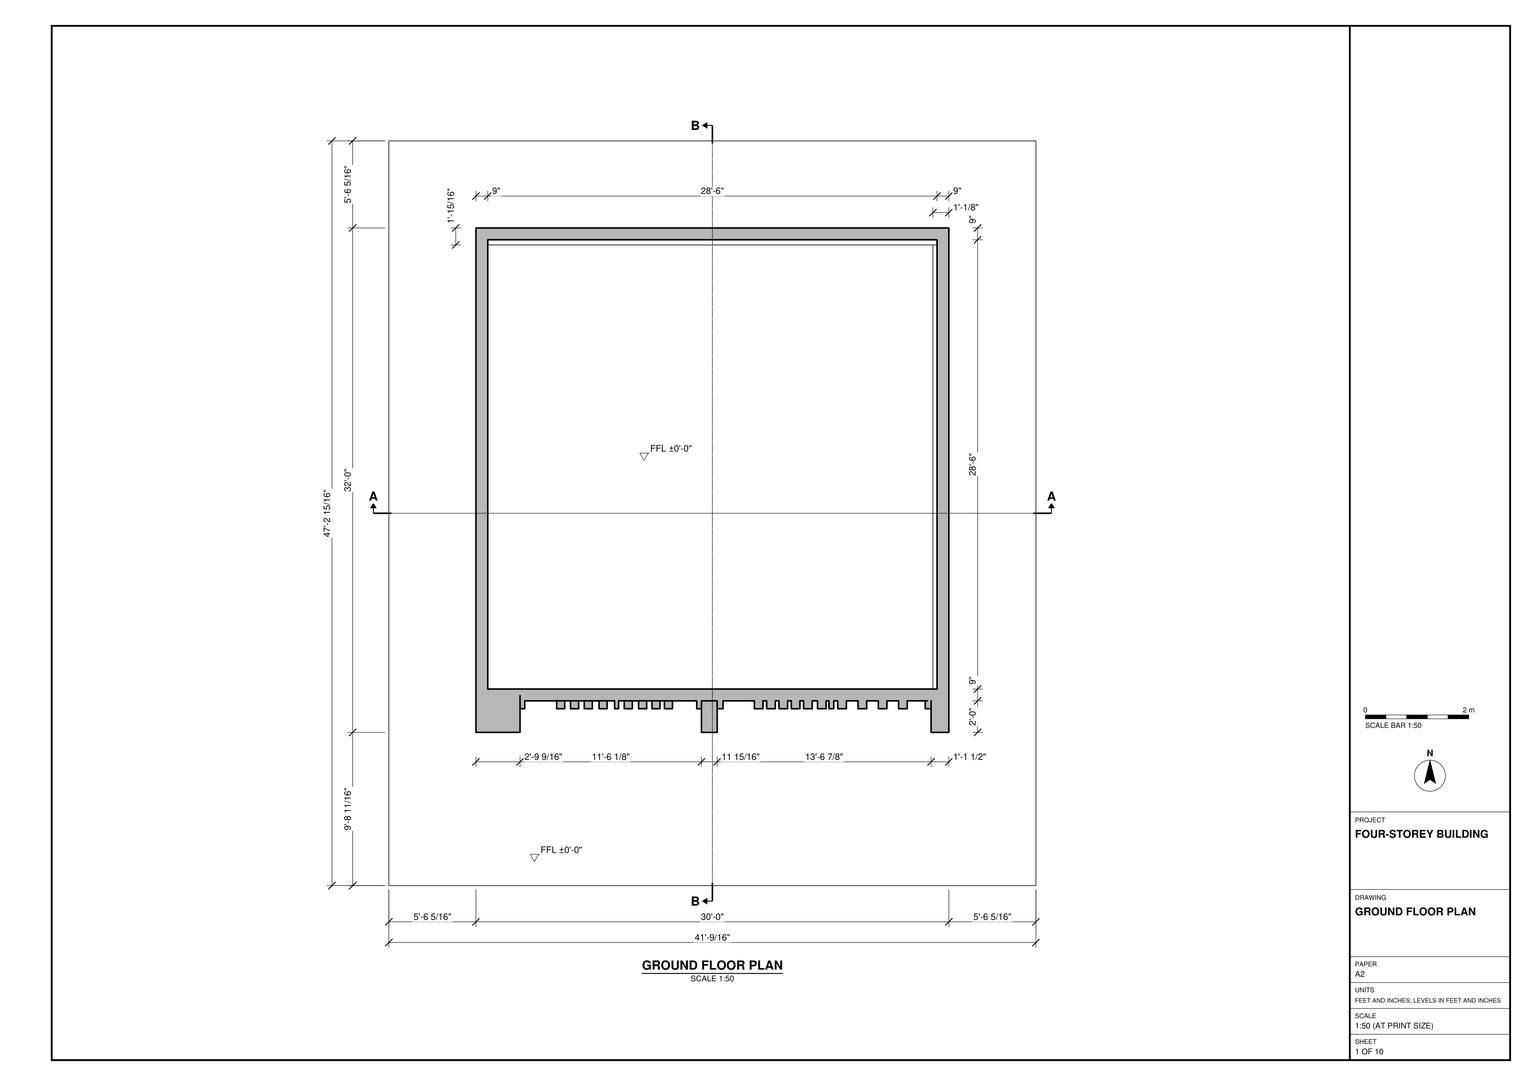
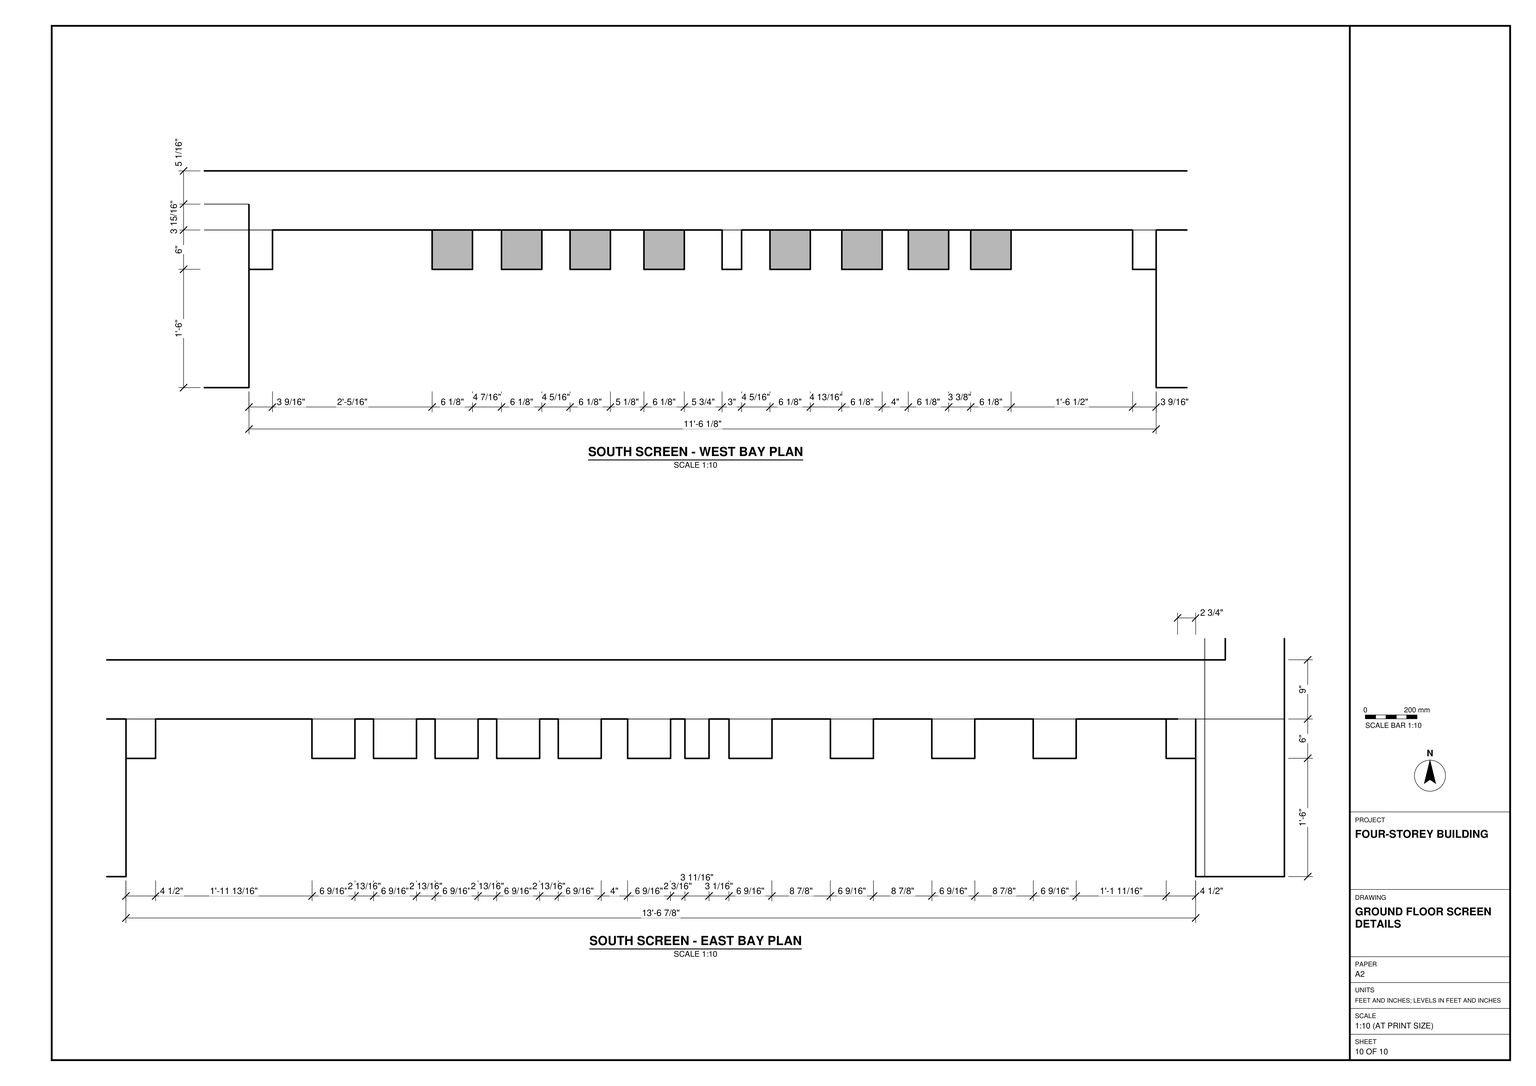
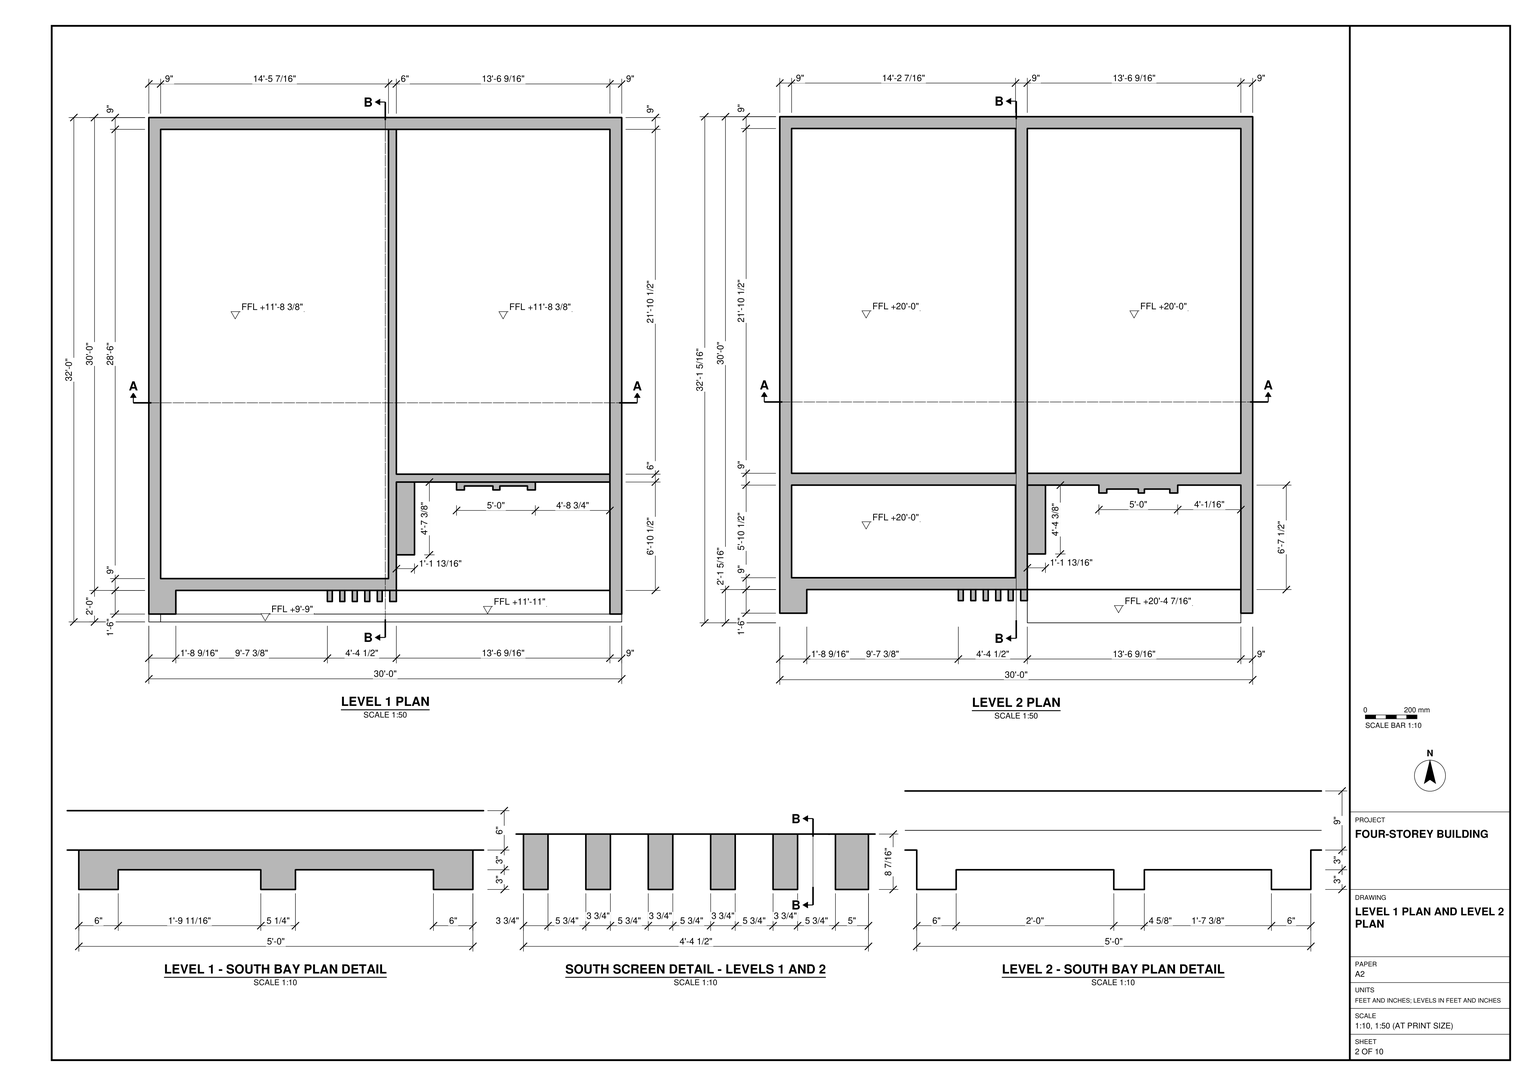
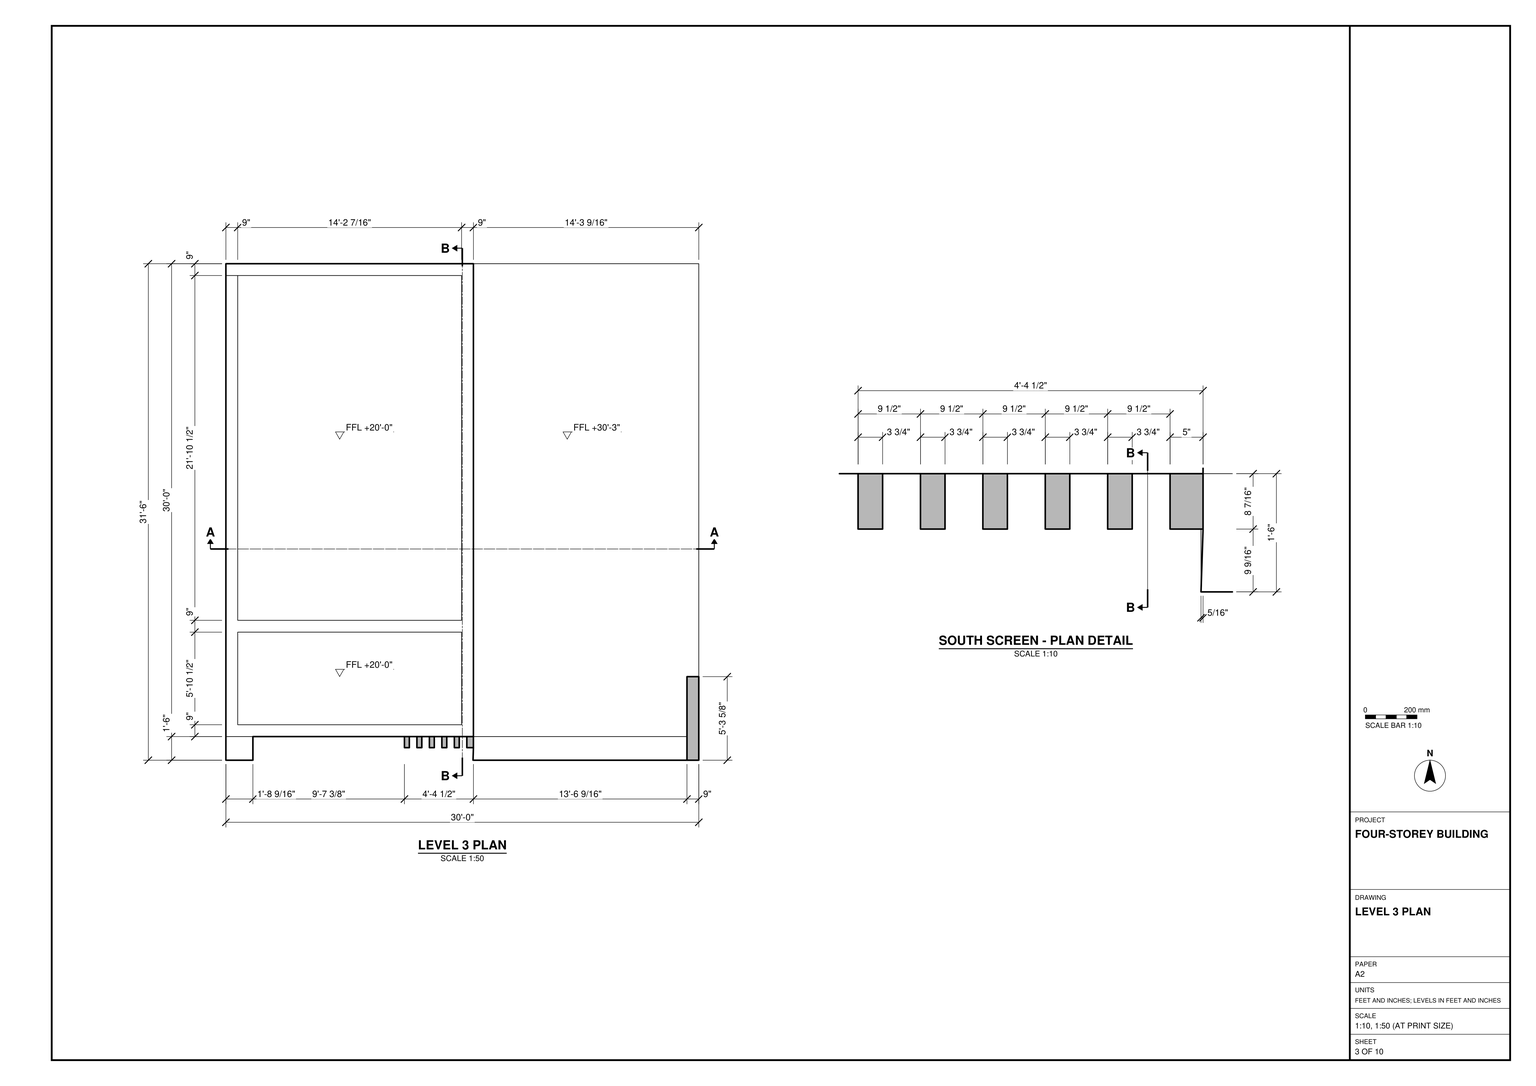
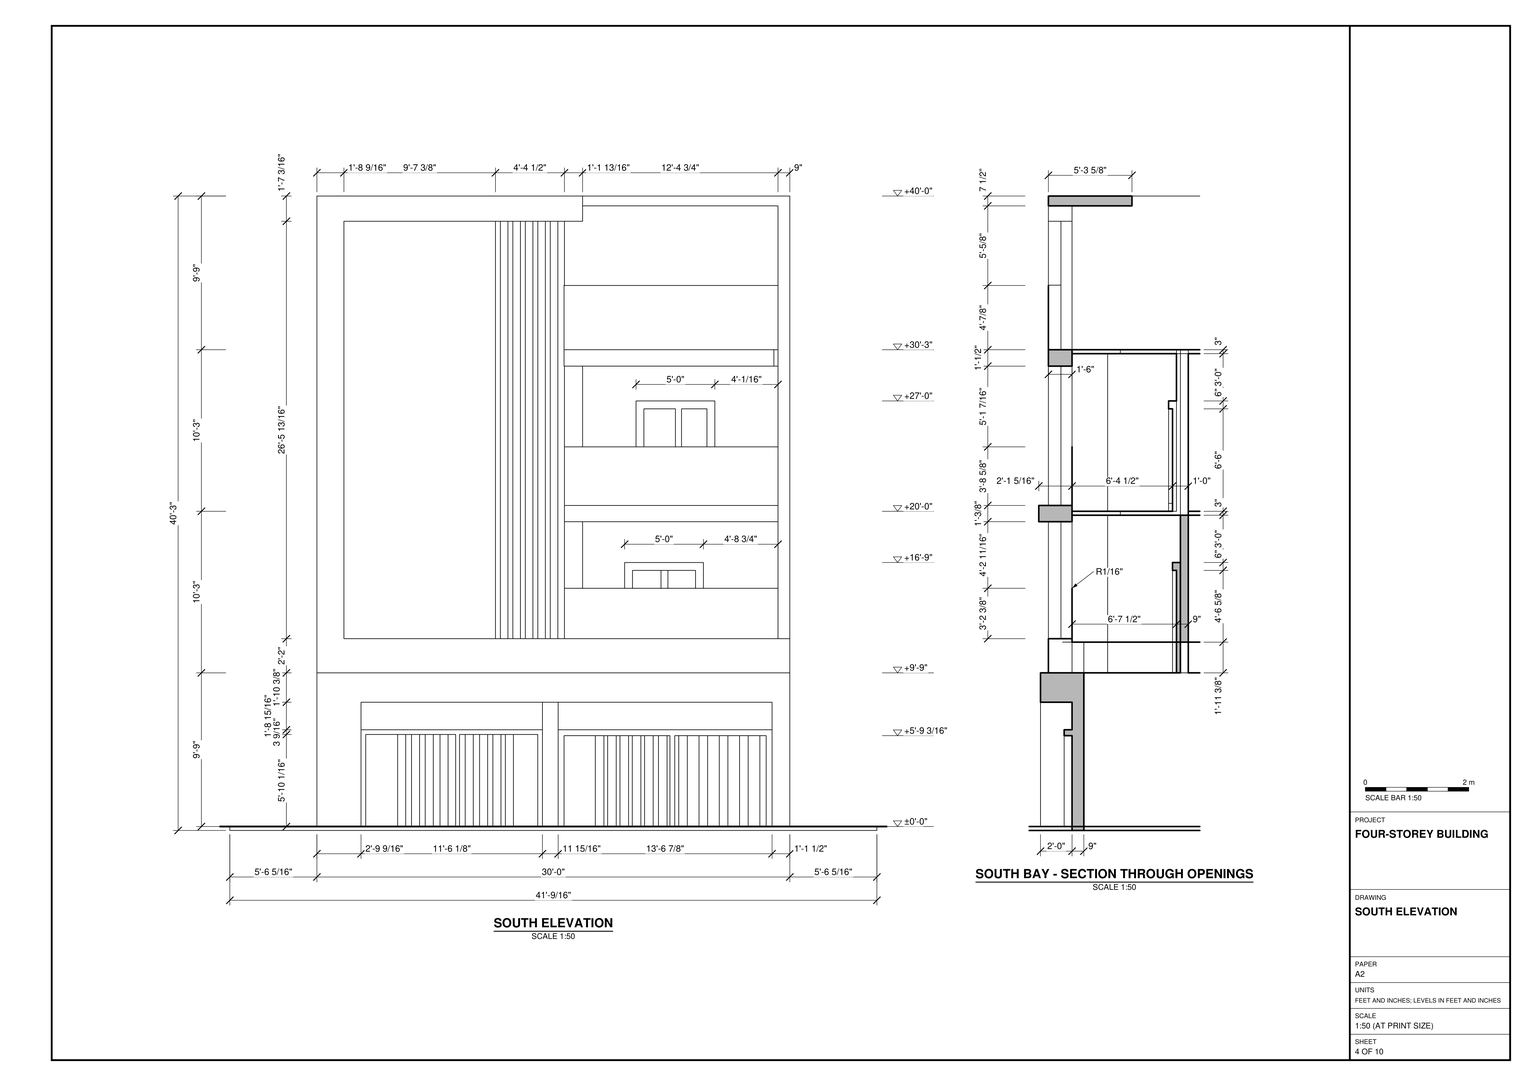
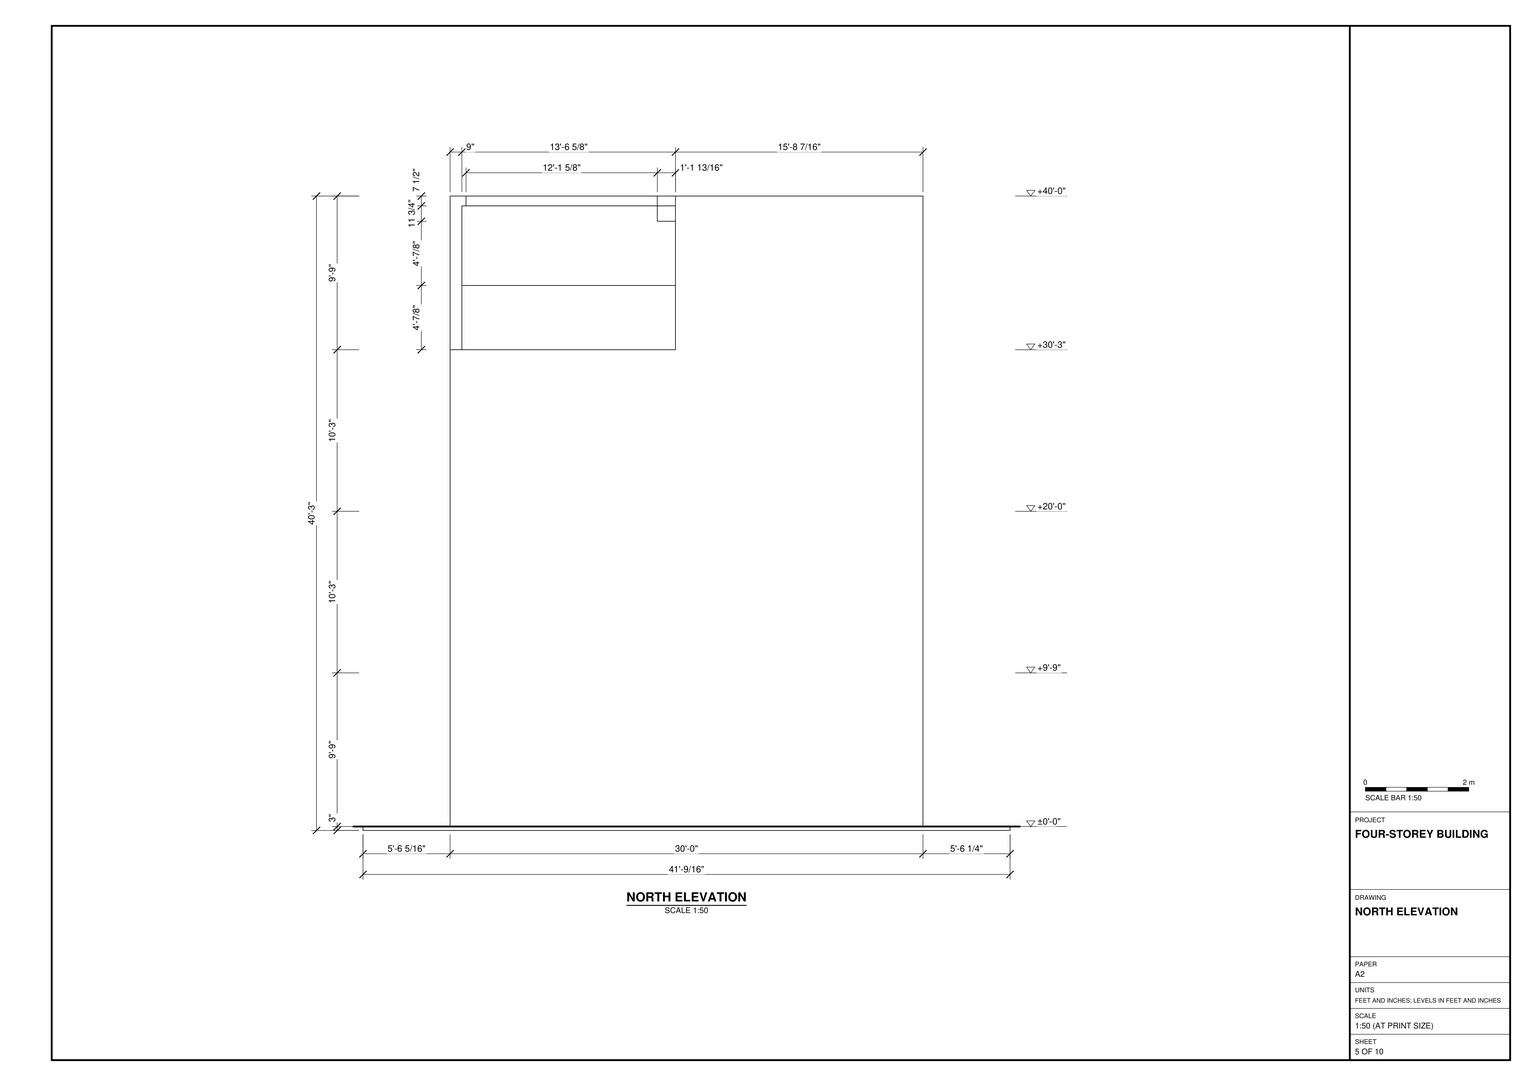
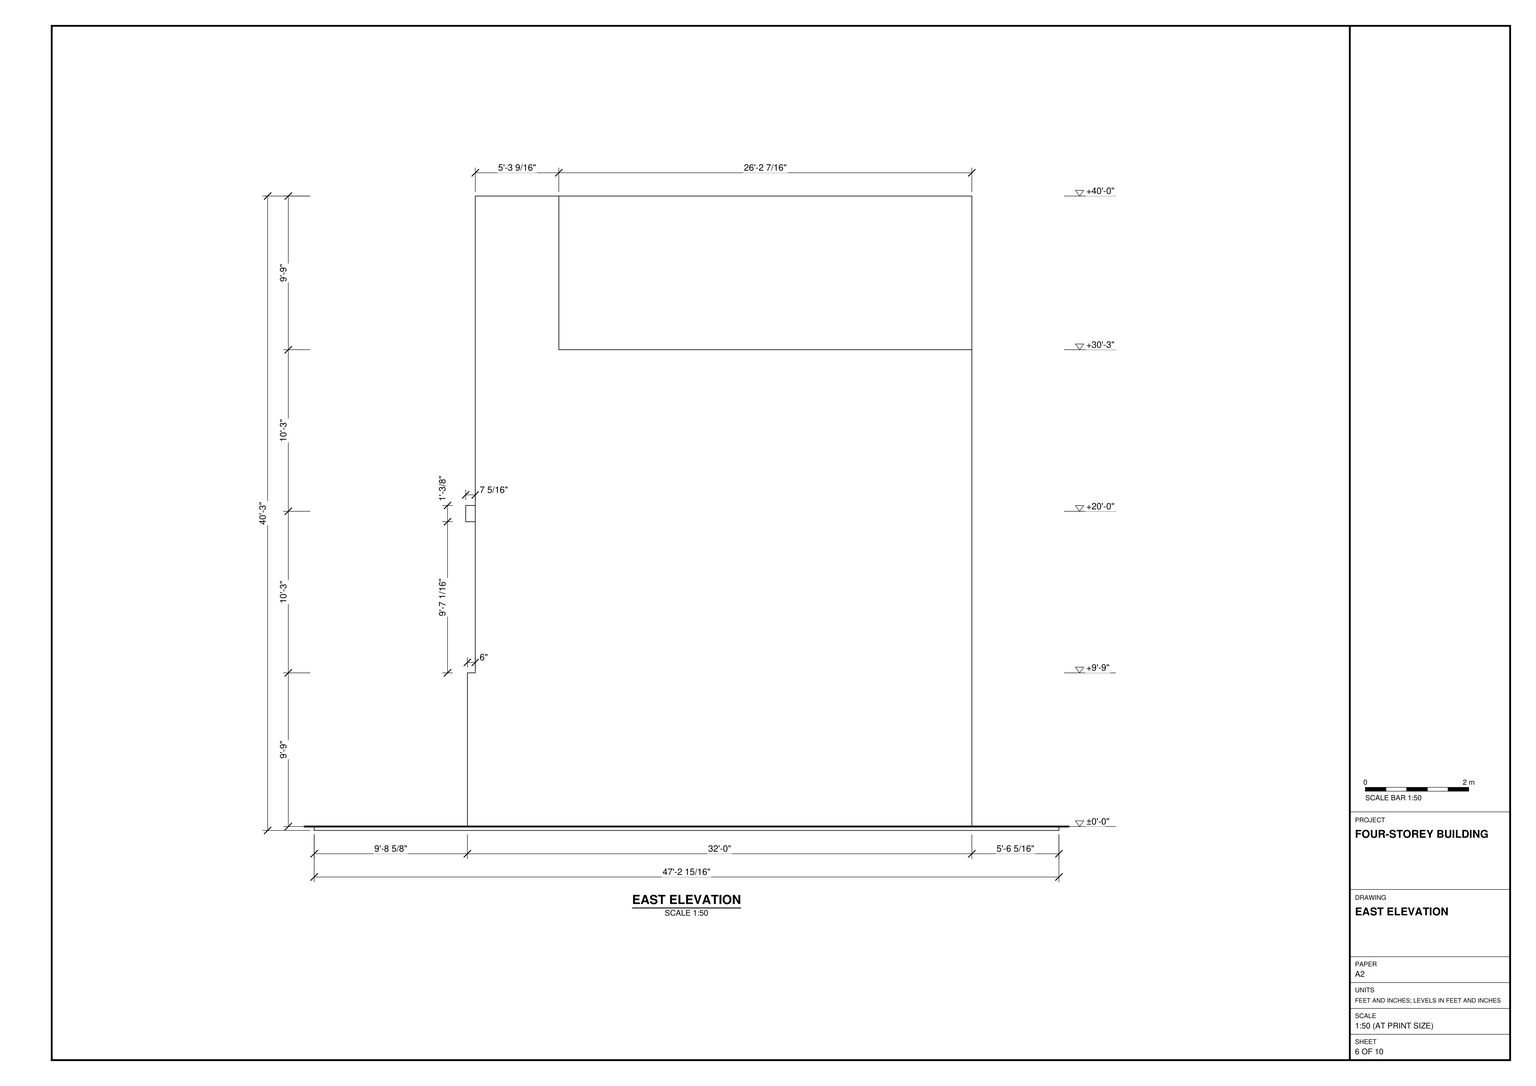
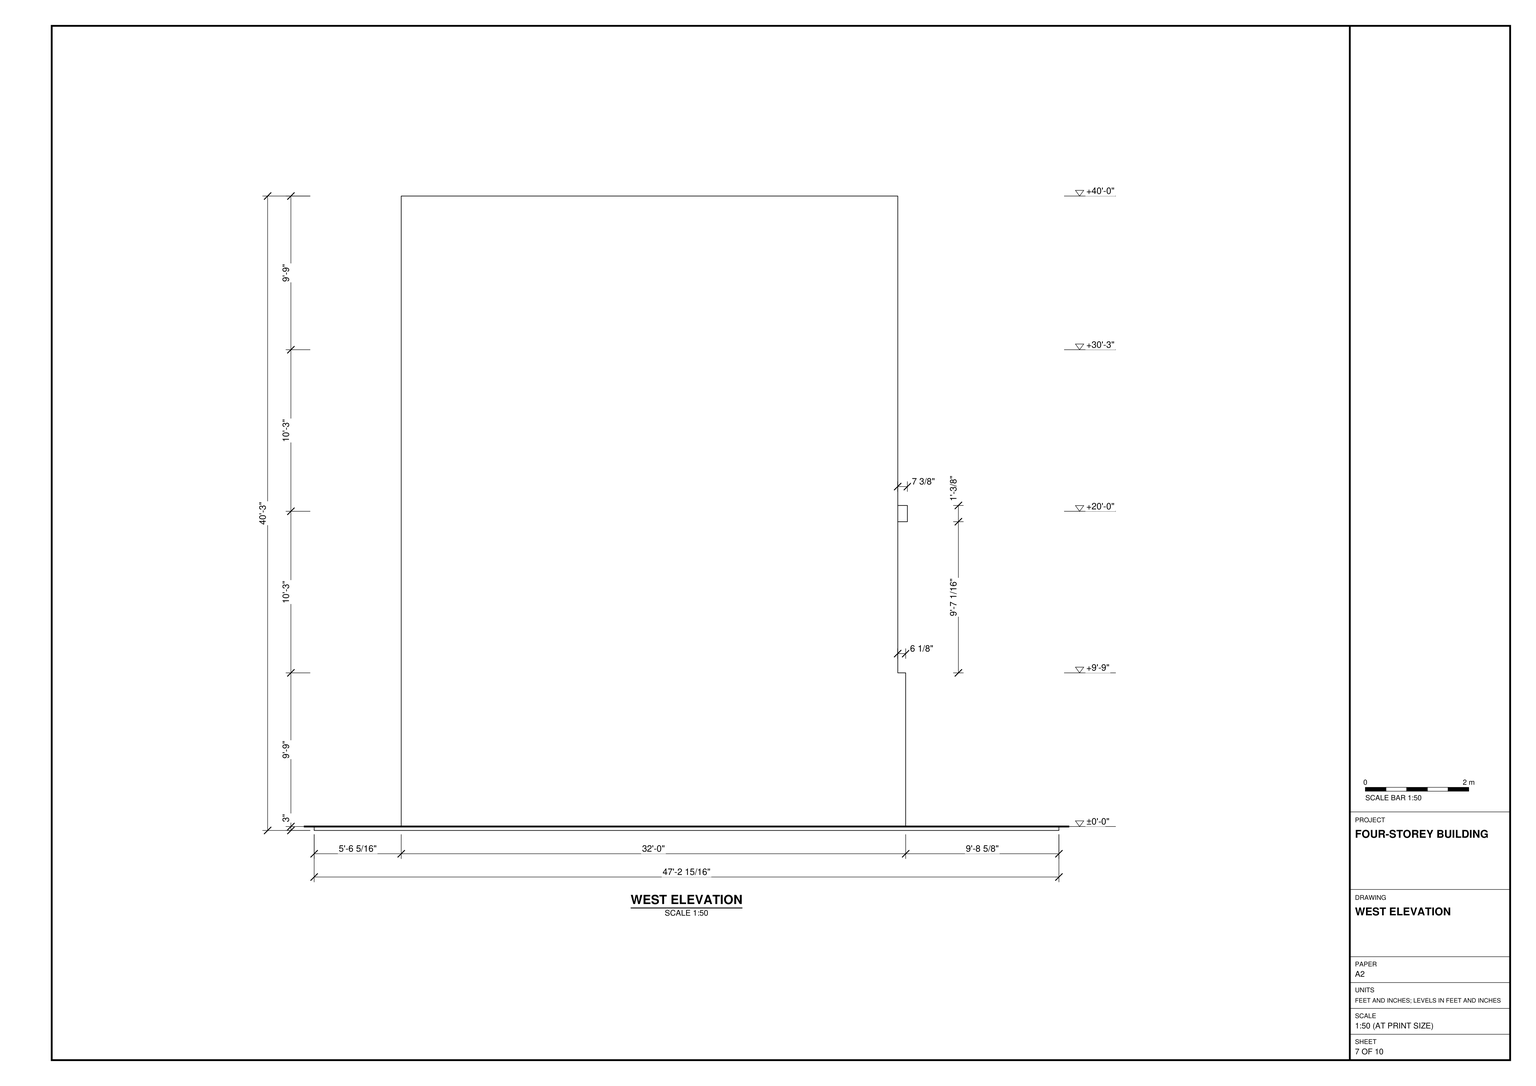
Build the four-storey building and its rectangular site in SketchUp using task_files/diagram_01.pdf. Work in feet and inches. The overall model measures 41'-9/16" east to west, 47'-2 15/16" north to south and 40'-3" high. Set out the storeys at ±0'-0", +9'-9", +20'-0" and +30'-3". Follow the local finished floor levels on the plans where a room or south bay differs from its storey reference level.

Place the building between the equal side margins, with the larger setback to the south. Model the open ground-floor interior, the perimeter walls and the projecting piers that frame the two unequal south screen bays. Use the enlarged details for the widths, spacing and projection of the screen members. Follow each upper plan separately: the internal wall thicknesses and the divisions behind the south façade change between floors. Include the recessed bays and the narrow upper screens rather than treating the south wall as a flat face.

Use the plans, elevations and sections together to locate the slabs, door and window openings, and roof. Include stairs, built-in joinery and main furniture where drawn. Keep shell elements such as walls, slabs and roof, and each furniture or joinery piece, in separate groups or components; use components for repeated parts. Decor and loose items may be any suitable library components. Save one SketchUp model as output_files/four_storey_building_with_screened_south_facade.skp.

# SketchUp Ruby script. Lengths in inches.
U = 1.inch
M = Sketchup.active_model
def pt(a) = Geom::Point3d.new(a.map { |v| v * U })
def face(e, loops, mat)
  f = e.add_face(loops[0].map { |a| pt(a) })
  loops[1..].each { |l| e.add_face(l.map { |a| pt(a) }).erase! }
  f.material = f.back_material = mat if mat
  f
end
# faces: each face lists its corners as indices into pts; further lists are holes
def faces(e, pts, list, mat = nil) = list.each { |f| face(e, (f[0].is_a?(Array) ? f : [f]).map { |l| l.map { |i| pts[i] } }, mat) }
# xy, xz, yz: faces in a plane at the given z, y or x. An outline is a flat list of corners, or four numbers for a rectangle; further outlines are holes
def ring(l) = l.size == 4 ? [[l[0], l[1]], [l[2], l[1]], [l[2], l[3]], [l[0], l[3]]] : l.each_slice(2).to_a
def flat(e, list, mat, &to3) = list.each { |f| face(e, (f[0].is_a?(Array) ? f : [f]).map { |l| ring(l).map { |u, v| to3.(u, v) } }, mat) }
def xy(e, z, list, mat = nil) = flat(e, list, mat) { |x, y| [x, y, z] }
def xz(e, y, list, mat = nil) = flat(e, list, mat) { |x, z| [x, y, z] }
def yz(e, x, list, mat = nil) = flat(e, list, mat) { |y, z| [x, y, z] }
def lines(e, pts, list) = list.each { |a, b| e.add_line(pt(pts[a]), pt(pts[b])) }
# prism: a flat outline (further loops are holes) pulled along v
def prism(e, loops, v, mat = nil)
  f = face(e, loops, mat); d = Geom::Vector3d.new(v.map { |x| x * U })
  f.pushpull(f.normal.samedirection?(d) ? d.length : -d.length)
end
def box(e, o, s, mat = nil) = prism(e, [[o, [o[0] + s[0], o[1], o[2]], [o[0] + s[0], o[1] + s[1], o[2]], [o[0], o[1] + s[1], o[2]]]], [0, 0, s[2]], mat)
def at(x, y, z, deg = 0) = Geom::Transformation.translation(pt([x, y, z])) * Geom::Transformation.rotation(ORIGIN, Z_AXIS, deg.degrees)
def axes(o, x, y, z) = Geom::Transformation.new([*x, 0, *y, 0, *z, 0, *pt(o).to_a, 1])
def part(name) = M.definitions.add(name)
# library, detail: a bought-in or finely detailed component or shape, given as its bounding box
def library(name, o, s) = part(name).tap { |d| box(d.entities, o, s) }
def detail(e, o, s) = box(e.add_group.entities, o, s)
def put(e, d, t, mat = nil) = e.add_instance(d, t).tap { |i| i.material = mat if mat }
def group(e, t, mat = nil) = e.add_group.tap { |g| g.transformation = t; g.material = mat if mat }.entities
root = M.entities
M.materials.add("[0035_Tan]").color = [124, 107, 83]
M.materials.add("[Color A08]").color = [102, 0, 0]
M.materials.add("[Color B05]").color = [255, 63, 0]
M.materials.add("[Color M09]").color = [0, 0, 0]
M.materials.add("[Encaustic Tile Circular 01]").color = [123, 123, 122]
M.materials.add("[Terrazzo]").color = [81, 71, 37]
M.materials.add("[Tile Limestone Multi]").color = [199, 173, 118]
M.materials.add("[Translucent Glass Blue]").color = [20, 30, 48]
M.materials["[Translucent Glass Blue]"].alpha = 0.5
M.materials.add("[Translucent Glass Gray]").color = [76, 76, 76]
M.materials["[Translucent Glass Gray]"].alpha = 0.5
M.materials.add("[Water Stream Shallow]").color = [191, 187, 34]
M.materials.add("[Wood Bamboo]").color = [130, 77, 31]
xy(root,0,[[[0,0,492.56,566.94],[75.28,133.41,417.28,133.41,417.28,140.66,426.28,140.66,426.28,500.66,66.28,500.66,66.28,491.66,60.22,491.66,60.22,140.66,75.28,140.66]],[75.28,133.41,417.28,140.66],[60.22,140.66,66.28,149.66],[66.28,140.66,75.28,149.66],[75.28,140.66,414.16,149.66],
  [414.16,140.66,417.28,149.66],[417.28,140.66,426.28,487.72],[60.22,149.66,66.28,491.66],[66.28,149.66,75.28,487.72],[75.28,149.66,414.16,487.72],
  [414.16,149.66,417.28,487.72],[417.28,487.72,417.28,491.66,66.28,491.66,66.28,500.66,426.28,500.66,426.28,487.72],[66.28,487.72,75.28,491.66],[75.28,487.72,417.28,491.66]])
xy(root,3,[[66.28,116.66,75.28,140.66],[75.28,116.66,99.85,140.66],[237.97,116.66,249.92,140.66],[412.78,116.66,414.16,140.66],[414.16,116.66,426.28,140.66],
  [99.85,134.66,103.43,140.66],[127.74,134.66,133.88,140.66],[138.3,134.66,144.45,140.66],[148.74,134.66,154.88,140.66],[159.99,134.66,166.13,140.66],
  [171.88,134.66,174.86,140.66],[179.18,134.66,185.32,140.66],[190.11,134.66,196.26,140.66],[200.24,134.66,206.38,140.66],[209.74,134.66,215.88,140.66],
  [234.39,134.66,237.97,140.66],[249.92,134.66,254.41,140.66],[278.23,134.66,284.77,140.66],[287.6,134.66,294.14,140.66],[296.98,134.66,303.52,140.66],
  [306.35,134.66,312.89,140.66],[315.73,134.66,322.27,140.66],[326.29,134.66,332.83,140.66],[335.01,134.66,338.68,140.66],[341.73,134.66,348.27,140.66],
  [357.16,134.66,363.7,140.66],[372.6,134.66,379.14,140.66],[388.04,134.66,394.58,140.66],[408.28,134.66,412.78,140.66],[66.28,140.66,75.28,144.59],
  [99.85,140.66,414.16,140.66,414.16,487.72,66.28,487.72,66.28,144.59,99.85,144.59],[75.28,140.66,99.85,144.59],[414.16,140.66,426.28,487.72],[66.28,487.72,426.28,500.66]])
xy(root,3,[[[0,0,492.56,566.94],[66.28,116.66,66.28,500.66,426.28,500.66,426.28,116.66,412.78,116.66,412.78,134.66,408.28,134.66,408.28,140.66,394.58,140.66,394.58,134.66,388.04,134.66,388.04,140.66,379.14,140.66,379.14,134.66,372.6,134.66,372.6,140.66,363.7,140.66,363.7,134.66,357.16,134.66,357.16,140.66,348.27,140.66,348.27,134.66,341.73,134.66,341.73,140.66,338.68,140.66,338.68,134.66,335.01,134.66,335.01,140.66,332.83,140.66,332.83,134.66,326.29,134.66,326.29,140.66,322.27,140.66,322.27,134.66,315.73,134.66,315.73,140.66,312.89,140.66,312.89,134.66,306.35,134.66,306.35,140.66,303.52,140.66,303.52,134.66,296.98,134.66,296.98,140.66,294.14,140.66,294.14,134.66,287.6,134.66,287.6,140.66,284.77,140.66,284.77,134.66,278.23,134.66,278.23,140.66,254.41,140.66,254.41,134.66,249.92,134.66,249.92,116.66,237.97,116.66,237.97,134.66,234.39,134.66,234.39,140.66,215.88,140.66,215.88,134.66,209.74,134.66,209.74,140.66,206.38,140.66,206.38,134.66,200.24,134.66,200.24,140.66,196.26,140.66,196.26,134.66,190.11,134.66,190.11,140.66,185.32,140.66,185.32,134.66,179.18,134.66,179.18,140.66,174.86,140.66,174.86,134.66,171.88,134.66,171.88,140.66,166.13,140.66,166.13,134.66,159.99,134.66,159.99,140.66,154.88,140.66,154.88,134.66,148.74,134.66,148.74,140.66,144.45,140.66,144.45,134.66,138.3,134.66,138.3,140.66,133.88,140.66,133.88,134.66,127.74,134.66,127.74,140.66,103.43,140.66,103.43,134.66,99.85,134.66,99.85,116.66]]],"[Tile Limestone Multi]")
xy(root,72.18,[[254.41,134.66,278.23,140.66],[284.77,134.66,287.6,140.66],[294.14,134.66,296.98,140.66],[303.52,134.66,306.35,140.66],[312.89,134.66,315.73,140.66],
  [322.27,134.66,326.29,140.66],[332.83,134.66,335.01,140.66],[338.68,134.66,341.73,140.66],[348.27,134.66,357.16,140.66],[363.7,134.66,372.6,140.66],
  [379.14,134.66,388.04,140.66],[394.58,134.66,408.28,140.66]],"[Color A08]")
xy(root,73.09,[[127.74,134.66,133.88,140.66],[138.3,134.66,144.45,140.66],[148.74,134.66,154.88,140.66],[159.99,134.66,166.13,140.66],[179.18,134.66,185.32,140.66],
  [190.11,134.66,196.26,140.66],[200.24,134.66,206.38,140.66],[209.74,134.66,215.88,140.66]])
xy(root,73.09,[[103.43,134.66,127.74,140.66],[133.88,134.66,138.3,140.66],[144.45,134.66,148.74,140.66],[154.88,134.66,159.99,140.66],[166.13,134.66,171.88,140.66],
  [174.86,134.66,179.18,140.66],[185.32,134.66,190.11,140.66],[196.26,134.66,200.24,140.66],[206.38,134.66,209.74,140.66],[215.88,134.66,234.39,140.66]],"[Color A08]")
xy(root,76.68,[[99.85,134.66,237.97,140.66],[249.92,134.66,412.78,140.66]],"[Color A08]")
xy(root,97.63,[[237.97,116.66,249.92,134.66],[237.97,134.66,249.92,140.66]])
xy(root,97.63,[[99.85,116.66,237.97,140.66],[249.92,116.66,412.78,140.66]],"[Tile Limestone Multi]")
xy(root,120,[[66.28,116.66,75.28,122.66],[75.28,122.66,238.84,134.66],[238.84,122.66,248.72,134.66],[248.72,122.66,254.72,134.66],[254.72,122.66,417.28,134.66],
  [75.28,134.66,238.84,140.66],[238.84,134.66,248.72,140.66],[248.72,134.66,254.72,140.66],[254.72,134.66,417.28,140.66],[75.28,140.66,248.72,149.66],
  [254.72,140.66,417.28,149.66],[75.28,149.66,248.72,491.66],[254.72,149.66,417.28,149.66,417.28,223.16,360.52,223.16,360.52,217.16,354.52,217.16,354.52,220.16,333.5,220.16,333.5,217.16,328.23,217.16,328.23,220.16,306.52,220.16,306.52,217.16,300.52,217.16,300.52,223.16,268.53,223.16,268.53,167.76,254.72,167.76],[254.72,167.76,268.53,177.38],[254.72,177.38,268.53,223.16],
  [300.52,217.16,306.52,220.16],[328.23,217.16,333.5,217.16,333.5,220.16,360.52,220.16,360.52,223.16,300.52,223.16,300.52,220.16,328.23,220.16],[354.52,217.16,360.52,220.16],[254.72,229.16,417.28,491.66]])
xy(root,120,[[75.28,116.66,426.28,122.66]],"[Tile Limestone Multi]")
xy(root,143.375,[[248.72,133.41,254.72,149.66]])
xy(root,143.375,[[254.72,140.66,417.28,140.66,417.28,491.66,75.28,491.66,75.28,149.66,254.72,149.66]],"[Encaustic Tile Circular 01]")
xy(root,146,[[202.2,132.22,205.93,137.66],[211.7,132.22,215.43,137.66],[221.2,132.22,224.93,137.66],[230.7,132.22,234.43,137.66],[240.2,132.22,243.93,137.66],
  [249.7,132.22,254.72,140.66],[202.2,137.66,205.93,140.66],[211.7,137.66,215.43,140.66],[221.2,137.66,224.93,140.66],[230.7,137.66,234.43,140.66],
  [240.2,137.66,243.93,140.66]])
xy(root,146,[[86.84,122.66,417.28,122.66,417.28,140.66,254.72,140.66,254.72,132.22,249.7,132.22,249.7,140.66,243.93,140.66,243.93,132.22,240.2,132.22,240.2,140.66,234.43,140.66,234.43,132.22,230.7,132.22,230.7,140.66,224.93,140.66,224.93,132.22,221.2,132.22,221.2,140.66,215.43,140.66,215.43,132.22,211.7,132.22,211.7,140.66,205.93,140.66,205.93,132.22,202.2,132.22,202.2,140.66,86.84,140.66]],"[Wood Bamboo]")
xy(root,198,[[306.52,217.16,328.23,220.16],[333.5,217.16,354.52,220.16]],"[Color M09]")
xy(root,204,[[300.52,217.16,360.52,223.16]],"[Color M09]")
xy(root,235.0625,[[254.72,115.34,417.28,140.66]],"[Wood Bamboo]")
xy(root,240,[[75.28,149.66,248.72,229.16],[254.72,167.76,268.53,177.38],[254.72,177.38,268.53,223.16],[254.72,223.16,417.28,229.16],[75.28,229.16,248.72,491.66],
  [248.72,229.16,254.72,491.66],[254.72,229.16,417.28,491.66]])
xy(root,240,[[254.72,140.66,254.72,167.76,268.53,167.76,268.53,223.16,417.28,223.16,417.28,140.66]],"[Water Stream Shallow]")
xy(root,243,[[75.28,149.66,245.72,220.16],[254.72,167.76,268.53,177.38],[254.72,177.38,268.53,220.16],[75.28,229.16,245.72,491.66],[254.72,229.16,417.28,491.66]])
xy(root,243,[[254.72,140.66,417.28,140.66,417.28,220.16,369.2,220.16,369.2,214.16,363.2,214.16,363.2,217.16,343.85,217.16,343.85,214.16,339.2,214.16,339.2,217.16,315.2,217.16,315.2,214.16,309.2,214.16,309.2,220.16,268.53,220.16,268.53,167.76,254.72,167.76]],"[Encaustic Tile Circular 01]")
xy(root,247.4375,[[254.72,115.34,417.28,140.66]],"[Wood Bamboo]")
xy(root,321,[[315.2,214.16,339.2,217.16],[343.85,214.16,363.2,217.16]],"[Color M09]")
xy(root,327,[[309.2,214.16,369.2,220.16]],"[Color M09]")
xy(root,353.5,[[254.41,122.66,254.41,132.22,254.72,132.22,254.72,140.66,417.28,140.66,417.28,122.66],[254.41,132.22,254.72,140.66]])
xy(root,363,[[254.72,167.76,268.53,177.38],[254.72,177.38,268.53,220.16],[254.72,229.16,417.28,491.66]])
xy(root,363,[[254.72,140.66,254.72,167.76,268.53,167.76,268.53,220.16,417.28,220.16,417.28,140.66]],"[Water Stream Shallow]")
xy(root,366,[[254.41,122.66,254.72,132.22,254.41,132.22],[254.41,122.66,417.28,122.66,417.28,140.66,254.72,140.66,254.72,132.22],[254.41,132.22,254.72,140.66],[254.72,140.66,417.28,140.66,417.28,186.28,426.28,186.28,426.28,500.66,254.72,500.66]])
xy(root,463.79,[[202.2,132.22,205.93,137.66],[211.7,132.22,215.43,137.66],[221.2,132.22,224.93,137.66],[230.7,132.22,234.43,137.66],[240.2,132.22,243.93,137.66],
  [249.7,132.22,254.72,140.66],[202.2,137.66,205.93,140.66],[211.7,137.66,215.43,140.66],[221.2,137.66,224.93,140.66],[230.7,137.66,234.43,140.66],
  [240.2,137.66,243.93,140.66]])
xy(root,463.79,[[86.84,122.66,86.84,140.66,202.2,140.66,202.2,132.22,205.93,132.22,205.93,140.66,211.7,140.66,211.7,132.22,215.43,132.22,215.43,140.66,221.2,140.66,221.2,132.22,224.93,132.22,224.93,140.66,230.7,140.66,230.7,132.22,234.43,132.22,234.43,140.66,240.2,140.66,240.2,132.22,243.93,132.22,243.93,140.66,249.7,140.66,249.7,132.22,254.72,132.22,254.72,140.66,268.53,140.66,268.53,122.66]],"[Wood Bamboo]")
xy(root,475.52,[[268.53,122.66,268.53,140.66,254.72,140.66,254.72,186.28,417.28,186.28,417.28,122.66]])
xy(root,483,[[66.28,122.66,426.28,122.66,426.28,186.28,254.72,186.28,254.72,500.66,66.28,500.66]])
xz(root,0,[[0,0,492.56,3]])
xz(root,115.34,[[254.72,235.0625,417.28,247.4375]],"[Wood Bamboo]")
xz(root,116.66,[[66.28,3,99.85,3,99.85,97.63,412.78,97.63,412.78,3,426.28,3,426.28,120,66.28,120],[237.97,3,249.92,97.63]],"[Tile Limestone Multi]")
xz(root,122.66,[[417.28,146,426.28,146,426.28,483,268.53,483,268.53,475.52,417.28,475.52],[254.41,353.5,414.16,366],[414.16,353.5,417.28,366]])
xz(root,122.66,[[254.41,366,417.28,414.89]],"[Translucent Glass Gray]")
xz(root,122.66,[[66.28,120,426.28,120,426.28,146,86.84,146,86.84,463.79,268.53,463.79,268.53,483,66.28,483]],"[Wood Bamboo]")
xz(root,132.22,[[202.2,146,205.93,463.79],[211.7,146,215.43,463.79],[221.2,146,224.93,463.79],[230.7,146,234.43,463.79],[240.2,146,243.93,463.79],
  [249.7,146,254.72,146,254.72,353.5,254.41,353.5,254.41,366,254.72,366,254.72,463.79,249.7,463.79]],"[0035_Tan]")
xz(root,134.66,[[99.85,3,103.43,3,103.43,73.09,171.88,73.09,171.88,3,174.86,3,174.86,73.09,234.39,73.09,234.39,3,237.97,3,237.97,76.68,99.85,76.68],[249.92,3,254.41,3,254.41,72.18,335.01,72.18,335.01,3,338.68,3,338.68,72.18,408.28,72.18,408.28,3,412.78,3,412.78,76.68,249.92,76.68]],"[Color A08]")
xz(root,134.66,[[127.74,3,133.88,73.09],[138.3,3,144.45,73.09],[148.74,3,154.88,73.09],[159.99,3,166.13,73.09],[179.18,3,185.32,73.09],
  [190.11,3,196.26,73.09],[200.24,3,206.38,73.09],[209.74,3,215.88,73.09],[278.23,3,284.77,72.18],[287.6,3,294.14,72.18],
  [296.98,3,303.52,72.18],[306.35,3,312.89,72.18],[315.73,3,322.27,72.18],[326.29,3,332.83,72.18],[341.73,3,348.27,72.18],
  [357.16,3,363.7,72.18],[372.6,3,379.14,72.18],[388.04,3,394.58,72.18]],"[Color B05]")
xz(root,140.66,[[66.28,0,75.28,3],[75.28,0,414.16,0,414.16,3,408.28,3,408.28,0.75,234.39,2.97,231.72,3,75.28,3],[414.16,0,426.28,3],[408.28,0.75,408.28,3,234.39,3,234.39,2.97],[234.39,2.97,234.39,3,231.72,3],
  [127.74,3,133.88,73.09],[138.3,3,144.45,73.09],[148.74,3,154.88,73.09],[159.99,3,166.13,73.09],[179.18,3,185.32,73.09],
  [190.11,3,196.26,73.09],[200.24,3,206.38,73.09],[209.74,3,215.88,73.09],[237.97,3,249.92,97.63],[408.28,3,410.02,72.18],
  [238.84,120,254.72,146],[254.72,143.375,417.28,146],[202.2,146,205.93,463.79],[211.7,146,215.43,463.79],[221.2,146,224.93,463.79],
  [230.7,146,234.43,463.79],[240.2,146,243.93,463.79],[249.7,146,249.7,463.79,254.72,463.79,254.72,366,254.41,366,254.41,353.5,254.72,353.5,254.72,146],[254.72,235.0625,417.28,240],[254.72,240,417.28,243],
  [254.72,243,417.28,247.4375],[254.41,353.5,254.72,363],[254.72,353.5,417.28,363],[254.41,363,254.72,366],[254.72,363,417.28,366],
  [254.72,463.79,268.53,475.52]])
xz(root,140.66,[[103.43,3,127.74,73.09],[133.88,3,138.3,73.09],[144.45,3,148.74,73.09],[154.88,3,159.99,73.09],[166.13,3,171.88,73.09],
  [174.86,3,179.18,73.09],[185.32,3,190.11,73.09],[196.26,3,200.24,73.09],[206.38,3,209.74,73.09],[215.88,3,234.39,73.09],
  [254.41,3,278.23,72.18],[284.77,3,287.6,72.18],[294.14,3,296.98,72.18],[303.52,3,306.35,72.18],[312.89,3,315.73,72.18],
  [322.27,3,326.29,72.18],[332.83,3,335.01,72.18],[338.68,3,341.73,72.18],[348.27,3,357.16,72.18],[363.7,3,372.6,72.18],
  [379.14,3,388.04,72.18],[394.58,3,403.48,72.18],[403.48,3,408.28,72.18]],"[Color A08]")
xz(root,140.66,[[86.84,146,202.2,463.79],[205.93,146,211.7,463.79],[215.43,146,221.2,463.79],[224.93,146,230.7,463.79],[234.43,146,240.2,463.79],
  [243.93,146,249.7,463.79]],"[Terrazzo]")
xz(root,140.66,[[99.85,76.68,237.97,97.63],[249.92,76.68,412.78,97.63]],"[Tile Limestone Multi]")
xz(root,140.66,[[254.72,146,417.28,184.36],[254.72,247.4375,417.28,292.04]],"[Translucent Glass Gray]")
xz(root,149.66,[[75.28,0,75.28,120,248.72,120,248.72,143.375,254.72,143.375,254.72,120,417.28,120,417.28,0],[75.28,120,248.72,143.375],[75.28,143.375,248.72,240],[75.28,243,245.72,363]])
xz(root,167.76,[[254.72,120,268.53,240],[254.72,243,268.53,363]],"[Water Stream Shallow]")
xz(root,186.28,[[417.28,366,417.28,475.52,414.16,475.52,414.16,483,426.28,483,426.28,366],[254.72,475.52,268.53,483],[268.53,475.52,414.16,483]])
xz(root,214.16,[[309.2,243,315.2,243,315.2,321,339.2,321,339.2,243,343.85,243,343.85,321,363.2,321,363.2,243,369.2,243,369.2,327,309.2,327]],"[Color M09]")
xz(root,217.16,[[300.52,120,306.52,120,306.52,198,354.52,198,354.52,120,360.52,120,360.52,204,300.52,204],[328.23,120,333.5,198]],"[Color M09]")
xz(root,217.16,[[315.2,243,339.2,321],[343.85,243,363.2,321]],"[Translucent Glass Blue]")
xz(root,220.16,[[75.28,243,245.72,363],[254.72,243,268.53,363]])
xz(root,220.16,[[306.52,120,328.23,198],[333.5,120,354.52,198]],"[Translucent Glass Blue]")
xz(root,220.16,[[268.53,243,309.2,243,309.2,327,369.2,327,369.2,243,417.28,243,417.28,363,268.53,363]],"[Water Stream Shallow]")
xz(root,223.16,[[254.72,120,268.53,240],[300.52,120,360.52,204]])
xz(root,223.16,[[268.53,120,300.52,120,300.52,204,360.52,204,360.52,120,417.28,120,417.28,240,268.53,240]],"[Water Stream Shallow]")
xz(root,229.16,[[254.72,120,417.28,240],[254.72,240,417.28,243],[75.28,243,245.72,363],[254.72,243,417.28,363]])
xz(root,487.72,[[66.28,0,414.16,3],[414.16,0,426.28,3]])
xz(root,491.66,[[75.28,0,417.28,120],[75.28,120,248.72,143.375],[248.72,120,254.72,143.375],[254.72,120,417.28,143.375],[75.28,143.375,248.72,240],
  [248.72,143.375,254.72,240],[254.72,143.375,417.28,240],[254.72,240,417.28,243],[75.28,243,245.72,363],[254.72,243,417.28,363]])
xz(root,500.66,[[66.28,0,426.28,3],[66.28,3,66.28,483,254.72,483,254.72,366,426.28,366,426.28,3]])
xz(root,566.94,[[0,0,492.56,3]])
yz(root,0,[[0,0,566.94,3]])
yz(root,66.28,[[487.72,0,500.66,3],[116.66,3,116.66,120,122.66,120,122.66,483,500.66,483,500.66,3]])
yz(root,75.28,[[149.66,0,491.66,120],[149.66,120,491.66,143.375],[149.66,143.375,491.66,240],[149.66,243,220.16,363],[229.16,243,482.66,363],
  [482.66,243,491.66,363]])
yz(root,86.84,[[122.66,146,140.66,463.79]],"[Wood Bamboo]")
yz(root,99.85,[[134.66,3,140.66,76.68],[140.66,3,144.59,76.68],[140.66,76.68,144.59,97.63]])
yz(root,99.85,[[116.66,3,134.66,3,134.66,76.68,140.66,76.68,140.66,97.63,116.66,97.63]],"[Tile Limestone Multi]")
yz(root,103.43,[[134.66,3,140.66,73.09]],"[Color A08]")
yz(root,127.74,[[134.66,3,140.66,73.09]],"[Color B05]")
yz(root,133.88,[[134.66,3,140.66,73.09]],"[Color B05]")
yz(root,138.3,[[134.66,3,140.66,73.09]],"[Color B05]")
yz(root,144.45,[[134.66,3,140.66,73.09]],"[Color B05]")
yz(root,148.74,[[134.66,3,140.66,73.09]],"[Color B05]")
yz(root,154.88,[[134.66,3,140.66,73.09]],"[Color B05]")
yz(root,159.99,[[134.66,3,140.66,73.09]],"[Color B05]")
yz(root,166.13,[[134.66,3,140.66,73.09]],"[Color B05]")
yz(root,171.88,[[134.66,3,140.66,73.09]],"[Color A08]")
yz(root,174.86,[[134.66,3,140.66,73.09]],"[Color A08]")
yz(root,179.18,[[134.66,3,140.66,73.09]],"[Color B05]")
yz(root,185.32,[[134.66,3,140.66,73.09]],"[Color B05]")
yz(root,190.11,[[134.66,3,140.66,73.09]],"[Color B05]")
yz(root,196.26,[[134.66,3,140.66,73.09]],"[Color B05]")
yz(root,200.24,[[134.66,3,140.66,73.09]],"[Color B05]")
yz(root,202.2,[[132.22,146,140.66,463.79]],"[0035_Tan]")
yz(root,205.93,[[132.22,146,140.66,463.79]],"[0035_Tan]")
yz(root,206.38,[[134.66,3,140.66,73.09]],"[Color B05]")
yz(root,209.74,[[134.66,3,140.66,73.09]],"[Color B05]")
yz(root,211.7,[[132.22,146,140.66,463.79]],"[0035_Tan]")
yz(root,215.43,[[132.22,146,140.66,463.79]],"[0035_Tan]")
yz(root,215.88,[[134.66,3,140.66,73.09]],"[Color B05]")
yz(root,221.2,[[132.22,146,140.66,463.79]],"[0035_Tan]")
yz(root,224.93,[[132.22,146,140.66,463.79]],"[0035_Tan]")
yz(root,230.7,[[132.22,146,140.66,463.79]],"[0035_Tan]")
yz(root,234.39,[[134.66,3,140.66,73.09]],"[Color A08]")
yz(root,234.43,[[132.22,146,140.66,463.79]],"[0035_Tan]")
yz(root,237.97,[[134.66,3,140.66,76.68]])
yz(root,237.97,[[116.66,3,116.66,97.63,140.66,97.63,140.66,76.68,134.66,76.68,134.66,3]],"[Tile Limestone Multi]")
yz(root,240.2,[[132.22,146,140.66,463.79]],"[0035_Tan]")
yz(root,243.93,[[132.22,146,140.66,463.79]],"[0035_Tan]")
yz(root,245.72,[[149.66,243,220.16,363],[229.16,243,491.66,363]])
yz(root,248.72,[[149.66,120,491.66,240]])
yz(root,249.7,[[132.22,146,140.66,463.79]],"[0035_Tan]")
yz(root,249.92,[[134.66,3,140.66,76.68]])
yz(root,249.92,[[116.66,3,134.66,3,134.66,76.68,140.66,76.68,140.66,97.63,116.66,97.63]],"[Tile Limestone Multi]")
yz(root,254.41,[[122.66,353.5,132.22,366],[132.22,353.5,140.66,363],[132.22,363,140.66,366]])
yz(root,254.41,[[134.66,3,140.66,72.18]],"[Color A08]")
yz(root,254.72,[[140.66,120,149.66,143.375],[167.76,120,177.38,240],[177.38,120,223.16,240],[229.16,120,491.66,240],[132.22,146,140.66,146,140.66,184.33,140.64,184.33,140.63,184.34,140.61,184.35,140.6,184.36,140.6,184.38,140.59,184.39,140.6,184.41,140.6,184.43,140.61,184.4375,140.625,184.45,140.64,184.46,140.66,235.0625,132.22,235.0625],
  [140.64,184.33,140.66,184.33,140.64,184.46,140.625,184.45,140.61,184.4375,140.6,184.43,140.6,184.41,140.59,184.39,140.6,184.38,140.6,184.36,140.61,184.35,140.63,184.34],[140.68,184.34,140.69,184.34,140.7,184.35,140.71,184.37,140.72,184.38,140.72,184.41,140.71,184.43,140.7,184.44,140.6875,184.45,140.67,184.46,140.66,184.46],[132.22,235.0625,140.66,240],[132.22,240,140.66,243],[140.66,240,177.38,243],
  [177.38,240,223.16,240,223.16,363,220.16,363,220.16,243,177.38,243],[223.16,240,229.16,363],[229.16,240,491.66,243],[132.22,243,140.66,247.4375],[167.76,243,177.38,363],
  [177.38,243,220.16,363],[229.16,243,491.66,363],[132.22,247.4375,140.66,353.5],[140.66,363,177.38,366],[177.38,363,220.16,366],
  [220.16,363,223.16,366],[223.16,363,229.16,366],[229.16,363,491.66,366]])
yz(root,254.72,[[132.22,366,140.66,463.79]],"[0035_Tan]")
yz(root,254.72,[[149.66,120,167.76,120,167.76,240,140.66,240,140.66,184.46,140.67,184.46,140.6875,184.45,140.7,184.44,140.71,184.43,140.72,184.41,140.72,184.38,140.71,184.37,140.7,184.35,140.69,184.34,140.68,184.34,140.66,143.375,149.66,143.375],[140.66,243,167.76,363],[140.66,366,500.66,366,500.66,483,186.28,483,186.28,475.52,140.66,475.52]],"[Water Stream Shallow]")
yz(root,254.72,[[115.34,235.0625,132.22,247.4375]],"[Wood Bamboo]")
yz(root,268.53,[[167.76,120,223.16,240],[167.76,243,220.16,363]],"[Water Stream Shallow]")
yz(root,268.53,[[122.66,463.79,140.66,475.52]],"[Wood Bamboo]")
yz(root,278.23,[[134.66,3,140.66,72.18]],"[Color B05]")
yz(root,284.77,[[134.66,3,140.66,72.18]],"[Color B05]")
yz(root,287.6,[[134.66,3,140.66,72.18]],"[Color B05]")
yz(root,294.14,[[134.66,3,140.66,72.18]],"[Color B05]")
yz(root,296.98,[[134.66,3,140.66,72.18]],"[Color B05]")
yz(root,300.52,[[217.16,120,223.16,204]],"[Color M09]")
yz(root,303.52,[[134.66,3,140.66,72.18]],"[Color B05]")
yz(root,306.35,[[134.66,3,140.66,72.18]],"[Color B05]")
yz(root,306.52,[[217.16,120,220.16,198]],"[Color M09]")
yz(root,309.2,[[214.16,243,220.16,327]],"[Color M09]")
yz(root,312.89,[[134.66,3,140.66,72.18]],"[Color B05]")
yz(root,315.2,[[214.16,243,217.16,249]])
yz(root,315.2,[[214.16,249,217.16,321]],"[Color M09]")
yz(root,315.73,[[134.66,3,140.66,72.18]],"[Color B05]")
yz(root,322.27,[[134.66,3,140.66,72.18]],"[Color B05]")
yz(root,326.29,[[134.66,3,140.66,72.18]],"[Color B05]")
yz(root,328.23,[[217.16,120,220.16,198]],"[Color M09]")
yz(root,332.83,[[134.66,3,140.66,72.18]],"[Color B05]")
yz(root,333.5,[[217.16,120,220.16,198]],"[Color M09]")
yz(root,335.01,[[134.66,3,140.66,72.18]],"[Color A08]")
yz(root,338.68,[[134.66,3,140.66,72.18]],"[Color A08]")
yz(root,339.2,[[214.16,243,217.16,321]],"[Color M09]")
yz(root,341.73,[[134.66,3,140.66,72.18]],"[Color B05]")
yz(root,343.85,[[214.16,243,217.16,321]],"[Color M09]")
yz(root,348.27,[[134.66,3,140.66,72.18]],"[Color B05]")
yz(root,354.52,[[217.16,120,220.16,198]],"[Color M09]")
yz(root,357.16,[[134.66,3,140.66,72.18]],"[Color B05]")
yz(root,360.52,[[217.16,120,223.16,204]],"[Color M09]")
yz(root,363.2,[[214.16,243,217.16,249]])
yz(root,363.2,[[214.16,249,217.16,321]],"[Color M09]")
yz(root,363.7,[[134.66,3,140.66,72.18]],"[Color B05]")
yz(root,369.2,[[214.16,243,220.16,327]],"[Color M09]")
yz(root,372.6,[[134.66,3,140.66,72.18]],"[Color B05]")
yz(root,379.14,[[134.66,3,140.66,72.18]],"[Color B05]")
yz(root,388.04,[[134.66,3,140.66,72.18]],"[Color B05]")
yz(root,394.58,[[134.66,3,140.66,72.18]],"[Color B05]")
yz(root,408.28,[[134.66,3,140.66,72.18]],"[Color A08]")
yz(root,412.78,[[134.66,3,140.66,76.68]])
yz(root,412.78,[[116.66,3,116.66,97.63,140.66,97.63,140.66,76.68,134.66,76.68,134.66,3]],"[Tile Limestone Multi]")
yz(root,414.16,[[140.66,0,487.72,3]])
yz(root,417.28,[[149.66,0,491.66,0,491.66,120,229.16,120,229.16,143.375,223.16,143.375,223.16,120,149.66,120],[140.66,120,223.16,143.375],[229.16,120,491.66,143.375],[223.16,143.375,229.16,240],[229.16,143.375,491.66,240],
  [122.66,235.0625,140.66,240],[122.66,240,140.66,243],[229.16,240,491.66,243],[122.66,243,140.66,247.4375],[229.16,243,491.66,363],
  [122.66,353.5,140.66,366],[122.66,366,186.28,475.52]])
yz(root,417.28,[[140.66,143.375,140.66,146,122.66,146,122.66,235.0625,140.66,235.0625,140.66,240,149.66,240,149.66,143.375],[149.66,143.375,223.16,240],[140.66,243,220.16,363],[122.66,247.4375,140.66,353.5]],"[Water Stream Shallow]")
yz(root,417.28,[[115.34,235.0625,122.66,247.4375]],"[Wood Bamboo]")
yz(root,426.28,[[140.66,0,487.72,3],[487.72,0,500.66,3],[116.66,3,500.66,3,500.66,366,186.28,366,186.28,483,122.66,483,122.66,120,116.66,120]])
yz(root,492.56,[[0,0,566.94,3]])
# 23 loose lines left out
p = [[254.72,132.22,366],[254.41,122.66,366],[254.41,122.66,414.89],[254.41,122.66,415.14],[254.72,132.22,415.14]]
faces(root,p,[[0,1,2,3,4]])
